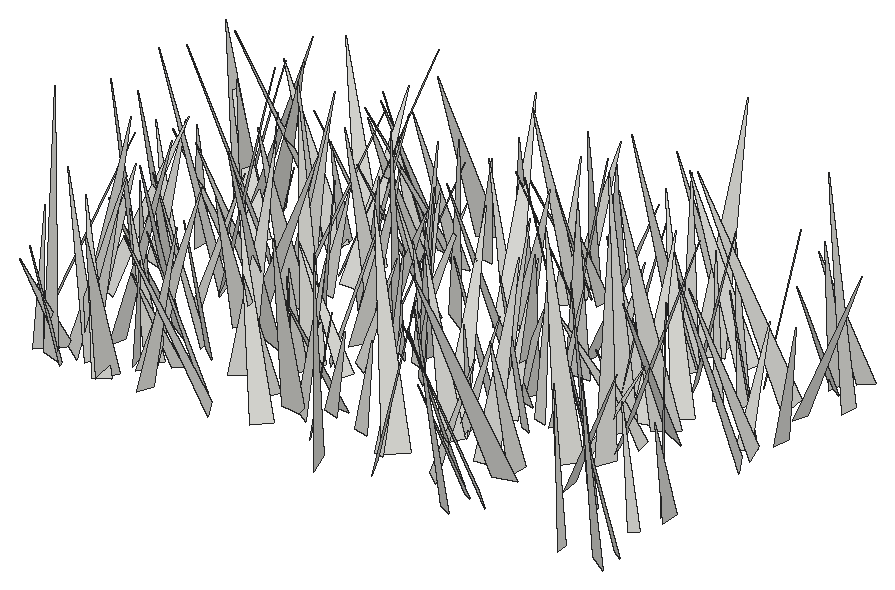
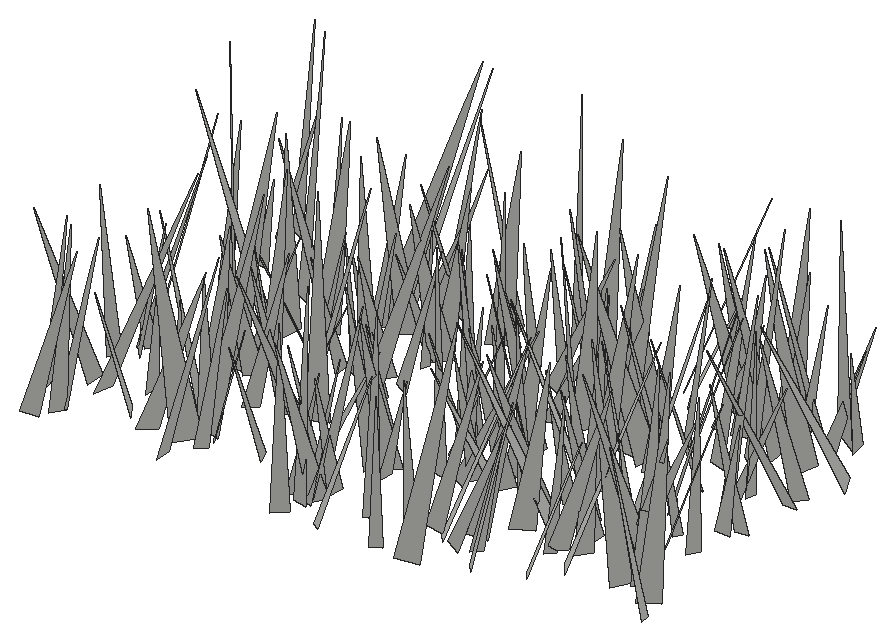
# SketchUp Ruby script. Lengths in inches.
U = 1.inch
M = Sketchup.active_model
def pt(a) = Geom::Point3d.new(a.map { |v| v * U })
def face(e, loops, mat)
  f = e.add_face(loops[0].map { |a| pt(a) })
  loops[1..].each { |l| e.add_face(l.map { |a| pt(a) }).erase! }
  f.material = f.back_material = mat if mat
  f
end
# faces: each face lists its corners as indices into pts; further lists are holes
def faces(e, pts, list, mat = nil) = list.each { |f| face(e, (f[0].is_a?(Array) ? f : [f]).map { |l| l.map { |i| pts[i] } }, mat) }
# xy, xz, yz: faces in a plane at the given z, y or x. An outline is a flat list of corners, or four numbers for a rectangle; further outlines are holes
def ring(l) = l.size == 4 ? [[l[0], l[1]], [l[2], l[1]], [l[2], l[3]], [l[0], l[3]]] : l.each_slice(2).to_a
def flat(e, list, mat, &to3) = list.each { |f| face(e, (f[0].is_a?(Array) ? f : [f]).map { |l| ring(l).map { |u, v| to3.(u, v) } }, mat) }
def xy(e, z, list, mat = nil) = flat(e, list, mat) { |x, y| [x, y, z] }
def xz(e, y, list, mat = nil) = flat(e, list, mat) { |x, z| [x, y, z] }
def yz(e, x, list, mat = nil) = flat(e, list, mat) { |y, z| [x, y, z] }
def lines(e, pts, list) = list.each { |a, b| e.add_line(pt(pts[a]), pt(pts[b])) }
# prism: a flat outline (further loops are holes) pulled along v
def prism(e, loops, v, mat = nil)
  f = face(e, loops, mat); d = Geom::Vector3d.new(v.map { |x| x * U })
  f.pushpull(f.normal.samedirection?(d) ? d.length : -d.length)
end
def box(e, o, s, mat = nil) = prism(e, [[o, [o[0] + s[0], o[1], o[2]], [o[0] + s[0], o[1] + s[1], o[2]], [o[0], o[1] + s[1], o[2]]]], [0, 0, s[2]], mat)
def at(x, y, z, deg = 0) = Geom::Transformation.translation(pt([x, y, z])) * Geom::Transformation.rotation(ORIGIN, Z_AXIS, deg.degrees)
def axes(o, x, y, z) = Geom::Transformation.new([*x, 0, *y, 0, *z, 0, *pt(o).to_a, 1])
def part(name) = M.definitions.add(name)
# library, detail: a bought-in or finely detailed component or shape, given as its bounding box
def library(name, o, s) = part(name).tap { |d| box(d.entities, o, s) }
def detail(e, o, s) = box(e.add_group.entities, o, s)
def put(e, d, t, mat = nil) = e.add_instance(d, t).tap { |i| i.material = mat if mat }
def group(e, t, mat = nil) = e.add_group.tap { |g| g.transformation = t; g.material = mat if mat }.entities
root = M.entities
c1 = part("fur_instance\#9")
p = [[0.8125,0,1.79],[0.67,-0.02,1.48],[0,-0.11,0],[0,0.11,0]]
faces(c1.entities,p,[[0,1,2,3]])
put(root,c1,axes([512.81,56.03,-21.66],[4.57924,-4.33247,0.58798],[-4.22206,-4.60304,-1.03525],[-1.13589,-0.35667,6.21836]))
put(root,c1,axes([519.8125,56.62,-21.66],[-5.72076,-3.26575,0.35826],[-3.1922,5.6955,0.94426],[0.77675,-0.64548,6.51924]))
put(root,c1,axes([528.72,55.54,-21.66],[6.72646,1.81373,2.96578],[2.30607,-7.16166,-0.85049],[-2.60144,-1.65881,6.91459]))
put(root,c1,axes([538.63,58.125,-21.66],[-4.50054,-5.78959,0.45114],[-5.68851,4.51005,1.13049],[1.1678,-0.3432,7.24542]))
put(root,c1,axes([548.48,56.47,-21.66],[-3.10043,-5.65859,2.0595],[-5.81568,3.41455,0.62657],[1.56175,1.48157,6.42182]))
put(root,c1,axes([508.82,57.23,-21.66],[1.51991,-3.61395,0.26794],[-3.4425,-1.53065,-1.11749],[-1.13207,-0.1975,3.75792]))
put(root,c1,axes([509.875,55.41,-21.66],[-3.12705,-1.8127,0.50032],[-1.87769,2.95706,-1.02213],[-0.10232,1.13341,3.46693]))
put(root,c1,axes([537.6875,55.89,-21.66],[-3.61019,-4.99925,2.09321],[-5.40705,3.49453,-0.97958],[0.37125,2.28107,6.08822]))
put(root,c1,axes([512.74,55.59,-21.66],[-2.01026,5.06538,1.49078],[5.275,1.85579,0.80751],[-0.23431,-1.67916,5.38954]))
put(root,c1,axes([515.45,56.19,-21.66],[5.24089,-0.83273,1.62957],[-1.05437,-5.41429,0.62423],[-1.49573,0.89885,5.2698]))
put(root,c1,axes([531.47,57.24,-21.66],[5.91305,2.63208,1.30513],[2.84881,-5.85376,-1.10147],[-0.71801,-1.54954,6.37799]))
put(root,c1,axes([508.86,55.72,-21.66],[2.99088,7.34321,2.70362],[7.47912,-3.53374,1.32409],[-2.30112,-1.94104,7.81761]))
put(root,c1,axes([545.77,56.53,-21.66],[-4.75488,-0.89522,1.48594],[-1.16705,4.85843,-0.80746],[1.28353,1.10117,4.77057]))
put(root,c1,axes([537.71,57.92,-21.66],[-2.11494,-3.26023,0.3236],[-3.25153,2.04149,-0.68318],[-0.40176,0.64034,3.82562]))
put(root,c1,axes([507.64,56.04,-21.66],[-4.10668,0.43412,1.0008],[0.12519,4.05996,-1.24738],[1.0837,1.17608,3.93666]))
put(root,c1,axes([509.49,56.92,-21.66],[3.29943,5.39851,1.49465],[5.593,-3.07886,-1.22601],[0.31023,-1.9081,6.20701]))
put(root,c1,axes([523.73,59.47,-21.66],[0.64901,-7.30772,0.94418],[-7.33385,-0.54888,0.79295],[0.71332,1.00569,7.2935]))
put(root,c1,axes([548.75,57.91,-21.66],[-3.27995,-3.84872,1.10692],[-4.00472,3.15616,-0.89264],[0.01123,1.42196,4.97734]))
put(root,c1,axes([513.13,58.27,-21.66],[3.69206,0.52175,1.19179],[0.74035,-3.79133,-0.63373],[-1.0698,-0.8231,3.6745]))
put(root,c1,axes([518.68,57.78,-21.66],[-4.50374,-2.5863,0.2222],[-2.55985,4.35118,-1.23954],[-0.43072,1.18335,5.04343]))
put(root,c1,axes([510.92,56.93,-21.66],[-5.72971,0.10944,0.75393],[-0.02545,5.68949,-1.01935],[0.7614,1.01378,5.63937]))
put(root,c1,axes([538.15,60.84,-21.66],[0.33917,-8.30019,0.61155],[-8.21231,-0.43312,-1.32383],[-1.35096,0.54903,8.20095]))
put(root,c1,axes([536.55,58.9,-21.66],[-2.94659,-4.28728,0.79485],[-4.35538,2.84813,-0.78348],[-0.2081,1.09651,5.14289]))
put(root,c1,axes([523.21,57.18,-21.66],[-3.60307,5.2202,0.86904],[5.28801,3.51043,0.83765],[-0.20649,-1.18922,6.28736]))
put(root,c1,axes([515.35,59.3125,-21.66],[0.6602,-3.48398,0.63366],[-3.31771,-0.83389,-1.12823],[-1.23791,0.37685,3.36171]))
put(root,c1,axes([513.87,59.01,-21.66],[2.18387,-4.44969,1.85832],[-4.59717,-2.53702,-0.67228],[-1.45572,1.33648,4.91091]))
put(root,c1,axes([526.45,57.6,-21.66],[2.93854,2.24557,1.05284],[2.03507,-3.11619,0.96641],[-1.41759,0.18132,3.56983]))
put(root,c1,axes([514.12,57.95,-21.66],[6.01682,-1.89651,1.60783],[-2.22,-5.99358,1.23799],[-1.11958,1.69241,6.18597]))
put(root,c1,axes([534.85,58.36,-21.66],[2.48119,3.58815,0.88423],[3.68479,-2.32113,-0.92071],[0.2811,-1.24521,4.2642]))
put(root,c1,axes([521.6,60.16,-21.66],[3.25434,-3.10316,1.28908],[-2.93626,-3.49873,-1.00964],[-1.63392,0.10675,4.38189]))
put(root,c1,axes([524.39,59.36,-21.66],[2.41252,4.65389,1.89869],[5.02303,-2.30836,-0.72433],[-0.1815,-2.02404,5.19175]))
put(root,c1,axes([528.28,59.95,-21.66],[0.50859,-3.54434,0.97529],[-3.61365,-0.30136,0.78924],[0.67458,1.05784,3.49258]))
put(root,c1,axes([525.55,60.61,-21.66],[0.50493,-3.90237,0.56248],[-3.75126,-0.30094,1.27958],[1.21364,0.69337,3.72104]))
put(root,c1,axes([530.68,58.56,-21.66],[1.32341,3.79294,0.4756],[3.74321,-1.38791,0.65276],[-0.77522,-0.22654,3.9638]))
put(root,c1,axes([525.92,61.32,-21.66],[-1.33885,-4.31341,0.19295],[-4.24788,1.27969,-0.86785],[-0.77346,0.43835,4.43226]))
put(root,c1,axes([531.43,59.28,-21.66],[-4.74257,5.72398,1.5327],[5.90767,4.72004,0.65254],[0.46105,-1.60076,7.40474]))
put(root,c1,axes([510.79,59.47,-21.66],[6.83211,0.09479,1.62922],[-0.11306,-6.96812,0.87954],[-1.62805,0.88169,6.77592]))
put(root,c1,axes([508.46,59.79,-21.66],[6.64236,-2.17739,2.19825],[-2.53423,-6.81539,0.90685],[-1.77512,1.5823,6.93106]))
put(root,c1,axes([512.82,62.5625,-21.66],[-2.64137,-6.46023,1.04071],[-6.35863,2.79897,1.23619],[1.54452,0.47506,6.86901]))
put(root,c1,axes([515.76,61.64,-21.66],[-2.72161,-4.19987,1.18368],[-4.18397,2.90781,0.69726],[1.23872,0.59401,4.95579]))
put(root,c1,axes([538.14,61.98,-21.66],[-4.48343,0.78051,2.64752],[1.64873,4.80743,1.37477],[2.21365,-1.99978,4.33824]))
put(root,c1,axes([543.55,62.14,-21.66],[-3.953,-6.85404,2.35159],[-6.87911,4.39144,1.23577],[2.27722,1.36799,7.81517]))
put(root,c1,axes([522.89,60.23,-21.66],[-3.3024,-1.44134,1.34219],[-1.74105,3.36144,-0.674],[0.92071,1.18661,3.53964]))
put(root,c1,axes([511.37,61.33,-21.66],[-4.43723,-6.45792,2.6794],[-6.95056,4.4181,-0.86196],[0.75734,2.71083,7.78786]))
put(root,c1,axes([548.45,63.11,-21.66],[4.29129,-1.7599,0.57931],[-1.53313,-4.1935,-1.38278],[-1.04037,-1.07949,4.42723]))
put(root,c1,axes([547.8,60.65,-21.66],[-0.43735,3.78387,0.74816],[3.7266,0.2203,1.06426],[-0.99494,-0.83814,3.65736]))
put(root,c1,axes([505.51,59.7,-21.66],[5.65943,2.62486,0.30549],[2.50558,-5.55953,1.3513],[-0.8398,1.10185,6.0904]))
put(root,c1,axes([541.65,62.45,-21.66],[5.27208,0.02621,0.0042],[0.02652,-5.23568,-0.61848],[-0.0011,-0.61849,5.23574]))
put(root,c1,axes([518.01,64.71,-21.66],[-1.4202,-8.16889,0.91065],[-8.13373,1.52988,1.03868],[1.18423,0.71114,8.22611]))
put(root,c1,axes([514.89,62.27,-21.66],[-5.1041,-1.8904,0.52095],[-1.9461,5.06157,-0.70004],[0.24022,0.83889,5.39772]))
put(root,c1,axes([521.18,63.26,-21.66],[3.43553,-2.13589,0.95207],[-2.02418,-3.56342,-0.68999],[-1.17096,-0.10667,3.98608]))
put(root,c1,axes([536.22,61.57,-21.66],[-1.99924,6.11191,2.2816],[6.3463,2.375,-0.80119],[1.51181,-1.88733,6.38047]))
put(root,c1,axes([518.68,60.92,-21.66],[5.55139,-3.03279,3.66915],[-4.09539,-5.91606,1.30628],[-2.42657,3.04644,6.18946]))
put(root,c1,axes([533.04,62.48,-21.66],[-4.86777,3.35697,1.6535],[3.6105,4.92638,0.62739],[0.98366,-1.46972,5.8797]))
put(root,c1,axes([506.51,62.82,-21.66],[2.49544,-4.2024,1.5625],[-4.46283,-2.15679,1.32672],[0.42981,2.0042,4.70396]))
put(root,c1,axes([547.34,63.79,-21.66],[6.08028,3.66314,2.96745],[4.34842,-6.22849,-1.22118],[-1.82087,-2.64225,6.99265]))
put(root,c1,axes([508.99,64.21,-21.66],[4.7247,0.27251,1.48983],[0.66278,-4.76043,-1.23114],[-1.36183,-1.37139,4.56961]))
put(root,c1,axes([533.07,63.99,-21.66],[3.93197,-0.07434,1.3447],[0.21137,-4.06439,-0.84276],[-1.33006,-0.86567,3.84131]))
put(root,c1,axes([515.14,65.55,-21.66],[4.0127,-3.86264,0.72099],[-3.71726,-4.06564,-1.09277],[-1.27351,-0.30356,5.46147]))
put(root,c1,axes([509.64,64.81,-21.66],[-1.12963,-3.6746,0.26296],[-3.62855,1.06225,-0.74377],[-0.63679,0.46567,3.77168]))
put(root,c1,axes([533.15,63.1,-21.66],[3.71678,-0.58843,1.31141],[-0.99782,-3.67326,1.17982],[-1.0346,1.42876,3.57333]))
put(root,c1,axes([523.51,64.55,-21.66],[-3.19624,2.75407,0.40141],[2.73336,2.9911,1.24258],[-0.52417,-1.19599,4.03198]))
put(root,c1,axes([539.93,64.58,-21.66],[-5.03128,5.10175,2.45438],[5.52933,5.13327,0.66454],[1.21582,-2.23324,7.13442]))
put(root,c1,axes([516.28,64.61,-21.66],[6.91635,-1.96319,0.7746],[-2.05636,-6.86586,0.95992],[-0.47486,1.1384,7.12521]))
put(root,c1,axes([532.75,62.86,-21.66],[-3.90742,5.66938,0.63215],[5.60395,3.95813,-0.85923],[1.06639,-0.02677,6.83166]))
put(root,c1,axes([521.38,64.19,-21.66],[-7.28379,2.71503,1.56111],[2.64145,7.44897,-0.63058],[1.68261,0.05921,7.74773]))
put(root,c1,axes([520.37,66.06,-21.66],[5.81902,2.09502,1.94943],[2.48849,-5.88572,-1.1028],[-1.4131,-1.7377,6.08555]))
put(root,c1,axes([506.48,63.76,-21.66],[1.55452,5.85258,0.28483],[5.77094,-1.47817,-1.12324],[1.01494,-0.55917,5.95042]))
put(root,c1,axes([539.57,65.29,-21.66],[1.87721,3.55983,2.07479],[3.45548,-2.60202,1.33802],[-2.2443,-1.02868,3.79553]))
put(root,c1,axes([511.88,65.3125,-21.66],[2.7927,4.03544,0.85961],[4.11922,-2.66751,-0.85986],[0.23622,-1.19268,4.83163]))
put(root,c1,axes([508.38,67.39,-21.66],[-2.6676,-6.3456,1.58153],[-6.4273,2.85927,0.63121],[1.20736,1.20081,6.85451]))
put(root,c1,axes([535.49,66.06,-21.66],[-2.59622,-3.87524,1.56211],[-4.17566,2.47102,-0.8099],[0.14666,1.75346,4.59368]))
put(root,c1,axes([523.5,65.8125,-21.66],[1.6531,3.56586,0.9383],[3.65871,-1.45863,-0.90264],[0.45784,-1.21883,3.82535]))
put(root,c1,axes([532.53,66.89,-21.66],[-2.18314,-4.32344,1.23175],[-4.48368,1.99494,-0.94459],[-0.32548,1.51774,4.75036]))
put(root,c1,axes([521.85,65.16,-21.66],[3.70568,3.40586,0.49894],[3.35111,-3.73706,0.62078],[-0.78668,0.12425,4.99466]))
put(root,c1,axes([541.56,65.85,-21.66],[-6.82221,1.72842,2.33339],[1.55801,7.20655,-0.7829],[2.45045,0.23004,6.99407]))
put(root,c1,axes([539.97,66.35,-21.66],[2.36408,2.77163,0.06713],[2.67068,-2.25294,-1.03299],[0.74428,-0.71945,3.49339]))
put(root,c1,axes([533.52,68.54,-21.66],[-2.92587,-7.18113,1.16279],[-7.26033,2.80394,-0.95233],[-0.45638,1.43204,7.69561]))
put(root,c1,axes([533.1875,69.09,-21.66],[6.03142,-3.81553,0.06105],[-3.78285,-5.99326,-0.84318],[-0.50203,-0.68018,7.08699]))
put(root,c1,axes([516.45,69.05,-21.66],[2.5513,-6.67742,1.15565],[-6.68995,-2.67869,-0.70836],[-1.08074,0.81812,7.11304]))
put(root,c1,axes([525.87,69.25,-21.66],[5.72206,-2.67718,0.30846],[-2.55509,-5.6197,-1.37653],[-0.85672,-1.12072,6.16558]))
put(root,c1,axes([525.14,66.66,-21.66],[-3.53887,0.08812,1.47041],[-0.2173,3.75324,-0.74791],[1.45693,0.77383,3.46005]))
put(root,c1,axes([541.94,68.82,-21.66],[-3.71284,-0.24914,0.82183],[0.046,3.58403,1.29433],[0.85753,-1.27095,3.48884]))
put(root,c1,axes([527.2,66.8,-21.66],[3.68214,4.39884,2.0354],[4.4735,-4.06815,0.69917],[-1.86561,-1.07294,5.69378]))
put(root,c1,axes([542.73,70.57,-21.66],[-1.67702,-6.45132,0.05531],[-6.32349,1.655,1.30744],[1.27907,-0.27646,6.53625]))
put(root,c1,axes([532.82,68.54,-21.66],[2.13927,-3.81253,0.27989],[-3.71667,-1.99926,1.17453],[0.89447,0.81104,4.21098]))
put(root,c1,axes([524.15,68.61,-21.66],[3.79237,5.90894,3.79832],[6.9076,-3.92109,-0.79686],[-1.27587,-3.6653,6.97586]))
put(root,c1,axes([533.98,66.38,-21.66],[-3.10832,3.75001,0.92239],[3.63037,3.24121,-0.94342],[1.31674,-0.08395,4.77852]))
put(root,c1,axes([511.85,67.94,-21.66],[-7.0839,-2.86843,1.00142],[-2.98784,7.03787,-0.97651],[0.55097,1.28563,7.57997]))
put(root,c1,axes([540.91,68.01,-21.66],[7.89024,2.57718,0.73013],[2.64489,-7.85516,-0.85554],[-0.42369,-1.04189,8.25626]))
put(root,c1,axes([535.51,67.33,-21.66],[1.56469,4.5597,1.40699],[4.65343,-1.78584,0.61247],[-1.05645,-1.11294,4.78163]))
put(root,c1,axes([521.78,67.87,-21.66],[5.79665,-1.91222,1.6292],[-2.17494,-5.87047,0.84811],[-1.25719,1.33905,6.04471]))
put(root,c1,axes([506.71,67.9,-21.66],[0.82444,4.69785,1.50621],[4.90559,-0.61872,-0.75536],[0.52313,-1.60174,4.70945]))
put(root,c1,axes([536.58,67.36,-21.66],[-4.01234,0.85775,1.7856],[0.34464,4.27421,-1.27879],[1.95072,1.00913,3.89863]))
put(root,c1,axes([547.68,70.55,-21.66],[-5.81163,-3.8947,1.27527],[-3.71182,5.94036,1.22659],[1.73708,-0.33677,6.88761]))
put(root,c1,axes([525.62,69.62,-21.66],[3.23004,-2.47849,1.2151],[-2.38486,-3.44753,-0.69249],[-1.3899,0.15559,4.01205]))
put(root,c1,axes([513.48,69.64,-21.66],[4.61843,1.91697,0.98697],[2.11588,-4.47821,-1.2031],[-0.41467,-1.49987,4.85358]))
put(root,c1,axes([507.57,68.6,-21.66],[-1.66438,3.94539,0.96796],[4.04045,1.49913,0.83702],[-0.42169,-1.20819,4.19948]))
put(root,c1,axes([526.01,68.07,-21.66],[2.58836,6.22661,1.98748],[6.38761,-2.86286,0.6503],[-1.38536,-1.56644,6.71174]))
put(root,c1,axes([511.66,67.93,-21.66],[6.24718,3.3719,1.68528],[3.2403,-6.4703,0.93425],[-1.92623,0.05148,7.03734]))
put(root,c1,axes([536.6875,69.58,-21.66],[-5.72763,-4.55632,1.57593],[-4.80185,5.61014,-1.23206],[0.43111,1.95337,7.21442]))
put(root,c1,axes([509.44,70.34,-21.66],[3.62629,-0.3933,0.08931],[-0.3696,-3.56406,-0.68808],[-0.16141,-0.67481,3.58206]))
put(root,c1,axes([520.99,70.77,-21.66],[1.6386,-6.2759,2.07036],[-6.47654,-1.94928,-0.78297],[-1.31443,1.78093,6.43885]))
put(root,c1,axes([541.84,71.04,-21.66],[2.92408,-7.38877,2.72238],[-7.56214,-3.44459,-1.22649],[-2.19528,2.02396,7.85111]))
put(root,c1,axes([511.32,70.93,-21.66],[-0.67131,-4.1889,0.93111],[-4.10147,0.34927,-1.38579],[-1.26165,1.09345,4.00962]))
put(root,c1,axes([547.5,72.07,-21.66],[-5.8236,-1.97497,1.08531],[-1.72724,5.8434,1.36532],[1.44743,-0.9731,5.99589]))
put(root,c1,axes([509.05,72.01,-21.66],[-4.05728,-2.523,0.42943],[-2.40041,4.03064,1.00168],[0.88766,-0.63233,4.67158]))
put(root,c1,axes([511.47,72.61,-21.66],[-5.81753,-5.50464,0.89808],[-5.45533,5.88597,0.73893],[1.16061,0.07452,7.97488]))
put(root,c1,axes([507.45,71.42,-21.66],[4.3427,-1.50818,1.19732],[-1.3579,-4.49272,-0.73402],[-1.36538,-0.32877,4.53816]))
put(root,c1,axes([540.08,69.5625,-21.66],[-7.50799,1.69583,1.59774],[1.55933,7.66276,-0.80567],[1.73121,0.45255,7.65484]))
put(root,c1,axes([525.82,70.52,-21.66],[-5.12979,-1.0122,0.11272],[-1.018,5.07872,-0.72273],[-0.03042,0.73083,5.17851]))
put(root,c1,axes([538.33,71.1,-21.66],[3.90059,1.73334,0.99556],[1.91928,-3.85762,-0.80331],[-0.55855,-1.15086,4.19211]))
put(root,c1,axes([516.6,71.29,-21.66],[-0.37702,3.57753,2.02822],[3.88687,0.97529,-0.99777],[1.34335,-1.81786,3.4562]))
put(root,c1,axes([520.51,72.17,-21.66],[3.4493,-3.36014,0.02886],[-3.29462,-3.37365,0.97621],[0.66096,0.719,4.71542]))
put(root,c1,axes([535.66,73.01,-21.66],[-3.34335,-1.51871,0.13226],[-1.40215,3.18862,1.16988],[0.59829,-1.01398,3.48078]))
put(root,c1,axes([533.93,72.84,-21.66],[1.85268,-6.56464,1.39244],[-6.70428,-1.74747,0.68181],[0.2934,1.52239,6.78691]))
put(root,c1,axes([518.4,73.18,-21.66],[5.40312,-1.02873,0.51523],[-0.87968,-5.28821,-1.33359],[-0.74156,-1.2223,5.33606]))
put(root,c1,axes([514.91,71.23,-21.66],[6.15209,3.35933,0.33959],[3.37614,-6.1107,-0.71393],[0.04606,-0.78923,6.97306]))
put(root,c1,axes([523.08,73.36,-21.66],[-1.88046,-5.21634,0.33238],[-5.10911,1.75978,-1.28722],[-1.10347,0.74146,5.39346]))
put(root,c1,axes([518.49,71.84,-21.66],[5.36031,4.39922,1.5205],[4.6383,-5.24227,-1.18439],[-0.38885,-1.88772,6.83252]))
put(root,c1,axes([530.55,70.43,-21.66],[1.48106,4.37962,0.44895],[4.22706,-1.54701,1.14671],[-1.23071,-0.04293,4.4788]))
put(root,c1,axes([524.4,73.45,-21.66],[-2.31612,-6.1908,2.36322],[-6.27799,2.85121,1.3163],[2.12077,1.67923,6.47748]))
put(root,c1,axes([522.84,72.18,-21.66],[2.35379,3.88662,0.95748],[3.9563,-2.09005,-1.24191],[0.60851,-1.44527,4.3708]))
put(root,c1,axes([514.25,72.32,-21.66],[4.29417,-2.87763,1.75823],[-3.19183,-4.38696,0.6155],[-1.08829,1.5119,5.13243]))
put(root,c1,axes([540.23,70.82,-21.66],[-3.17134,4.85922,0.78552],[4.77597,3.26378,-0.90795],[1.19131,-0.14895,5.73106]))
put(root,c1,axes([546.72,72.03,-21.66],[-2.21972,3.26489,1.22418],[3.2229,2.47495,-0.75684],[1.3308,-0.54808,3.87477]))
put(root,c1,axes([547.09,72.82,-21.66],[2.56501,3.25674,2.5986],[3.3721,-3.41499,0.95138],[-2.44704,-1.29222,4.03491]))
put(root,c1,axes([547.91,74.03,-21.66],[4.83385,-1.43847,0.54232],[-1.36908,-4.84202,-0.64023],[-0.69925,-0.46374,5.00254]))
put(root,c1,axes([522.52,72.52,-21.66],[-2.57998,2.99071,1.64125],[3.02202,2.95835,-0.64026],[1.58287,-0.77341,3.89753]))
put(root,c1,axes([538,73.875,-21.66],[-4.52682,2.09063,1.69581],[2.46981,4.54531,0.98938],[1.07078,-1.64562,4.88712]))
put(root,c1,axes([535.84,73.3,-21.66],[1.71183,-4.04593,1.56999],[-4.29437,-1.33542,1.2409],[0.62675,1.9005,4.21427]))
put(root,c1,axes([507.27,76.26,-21.66],[4.70982,-4.44224,0.12242],[-4.38661,-4.67586,-0.90827],[-0.71149,-0.57769,6.41023]))
put(root,c1,axes([541.74,72.7,-21.66],[-2.77056,6.19265,0.76015],[6.19361,2.62958,1.15202],[-0.75223,-1.15721,6.68563]))
put(root,c1,axes([512.31,75.42,-21.66],[5.42089,-2.3865,1.81758],[-2.19868,-5.71457,-0.94576],[-2.04078,-0.18248,5.84696]))
put(root,c1,axes([521.05,72.53,-21.66],[4.24517,2.47398,0.29086],[2.34061,-4.15824,1.20716],[-0.85248,0.90284,4.76286]))
put(root,c1,axes([512.71,73.75,-21.66],[5.08359,-0.28901,1.82683],[-0.68576,-5.25683,1.07667],[-1.71772,1.24337,4.97667]))
put(root,c1,axes([527.8,75.3,-21.66],[3.51302,-4.23345,1.0034],[-4.35037,-3.40123,0.88101],[0.05668,1.33409,5.43021]))
put(root,c1,axes([509.77,73.875,-21.66],[-3.53792,4.34861,0.23075],[4.30519,3.44804,1.02808],[-0.65501,-0.82532,5.51093]))
put(root,c1,axes([517.29,72.82,-21.66],[-1.69129,6.09931,0.73665],[6.01995,1.79783,-1.06428],[1.22654,-0.41345,6.23934]))
put(root,c1,axes([513.87,76.52,-21.66],[4.34393,-1.36952,0.92271],[-1.07858,-4.31928,-1.3331],[-1.25046,-1.03195,4.35524]))
put(root,c1,axes([508.99,75.42,-21.66],[3.83115,1.46002,1.29175],[1.69697,-3.89964,-0.62537],[-0.95945,-1.06731,4.05194]))
put(root,c1,axes([512.04,77.45,-21.66],[-5.96811,-4.81477,0.42538],[-4.75156,5.96808,0.88657],[0.88638,-0.42578,7.61672]))
put(root,c1,axes([508.34,76.93,-21.66],[6.88515,-2.28469,0.18682],[-2.24647,-6.84269,-0.88939],[-0.45618,-0.78602,7.19959]))
put(root,c1,axes([508.27,74.44,-21.66],[6.55283,1.12937,1.12544],[0.97488,-6.60494,0.95181],[-1.26162,0.76214,6.58096]))
put(root,c1,axes([518.27,77.71,-21.66],[1.50349,-5.86365,0.5049],[-5.82358,-1.55753,-0.74685],[-0.85041,0.2992,6.00709]))
put(root,c1,axes([540.07,75.82,-21.66],[5.73054,2.09287,1.0832],[2.24178,-5.71944,-0.8093],[-0.7265,-1.14039,6.04684]))
put(root,c1,axes([513.75,75.98,-21.66],[-5.32926,2.77314,1.19327],[2.9808,5.21718,1.1879],[0.47858,-1.6143,5.88899]))
put(root,c1,axes([505.83,77.55,-21.66],[4.78165,-4.93816,1.39024],[-4.88475,-4.96331,-0.82896],[-1.56762,0.40313,6.82367]))
put(root,c1,axes([533.17,74.86,-21.66],[5.62442,0.34622,0.61815],[0.22701,-5.5658,1.05184],[-0.67115,1.01884,5.53603]))
put(root,c1,axes([515.5625,74.09,-21.66],[6.75975,3.62956,0.52461],[3.54067,-6.74583,1.04905],[-0.95528,0.68056,7.60048]))
put(root,c1,axes([519.79,79.04,-21.66],[-4.86076,-4.47494,0.06756],[-4.36579,4.76306,1.38194],[0.98465,-0.972,6.46083]))
put(root,c1,axes([516.86,75.37,-21.66],[-4.60264,5.20733,0.96805],[5.29634,4.53648,0.77902],[0.04773,-1.24166,6.90606]))
put(root,c1,axes([545.83,77.65,-21.66],[-8.03194,-0.35365,0.82088],[-0.22203,7.97883,1.26494],[0.86581,-1.23463,7.93959]))
put(root,c1,axes([538.1,77.7,-21.66],[-1.48143,-7.59825,2.03928],[-7.84224,1.26126,-0.99758],[-0.62555,2.18232,7.67677]))
put(root,c1,axes([526.82,75.54,-21.66],[-4.67353,1.04438,0.03845],[1.02272,4.60667,-0.8165],[0.21505,0.78861,4.71868]))
put(root,c1,axes([543.59,75.95,-21.66],[-4.82421,0.67017,1.12309],[0.52178,4.9221,-0.69578],[1.19925,0.5543,4.82058]))
put(root,c1,axes([542.04,75.55,-21.66],[0.68638,4.30492,0.85677],[4.11958,-0.93113,1.37825],[-1.51508,-0.58153,4.13569]))
put(root,c1,axes([527.17,74.67,-21.66],[-3.85678,5.81728,0.33644],[5.7739,3.8696,-0.71896],[0.78484,0.11882,6.94252]))
put(root,c1,axes([530.33,77.85,-21.66],[-3.6362,-3.51378,0.23491],[-3.4583,3.49912,-1.19165],[-0.6648,1.01649,4.91412]))
put(root,c1,axes([520.81,78.5,-21.66],[-0.18696,-5.47828,1.21386],[-5.53827,-0.01495,-0.92048],[-0.90141,1.22808,5.40363]))
put(root,c1,axes([546.94,76.99,-21.66],[5.55155,-0.72144,0.45458],[-0.77671,-5.51397,0.73462],[-0.35191,0.78896,5.54982]))
put(root,c1,axes([513.29,79.41,-21.66],[-3.4189,-2.83051,0.24342],[-2.77437,3.40847,0.66713],[0.61145,-0.36118,4.38812]))
put(root,c1,axes([537.24,79.375,-21.66],[4.28198,-1.79299,1.3249],[-1.43721,-4.41332,-1.32759],[-1.70429,-0.78312,4.44833]))
put(root,c1,axes([537.33,78.05,-21.66],[-3.51582,-2.14374,0.80605],[-2.26912,3.46073,-0.69338],[0.31056,1.01688,4.05904]))
put(root,c1,axes([524.47,79.75,-21.66],[-0.27546,-6.0552,1.07535],[-6.00995,0.49341,1.23885],[1.30474,0.99438,5.93351]))
put(root,c1,axes([538.68,77.18,-21.66],[-5.6137,1.8249,1.28834],[1.63706,5.7317,-0.98561],[1.51991,0.56669,5.82001]))
put(root,c1,axes([517.29,79,-21.66],[-3.50463,1.38607,1.3282],[1.66931,3.56562,0.68373],[0.94799,-1.15452,3.70623]))
put(root,c1,axes([504.83,79.14,-21.66],[4.88196,1.64498,0.71636],[1.77456,-4.73338,-1.22423],[-0.26474,-1.39349,5.00407]))
put(root,c1,axes([546.35,80.79,-21.66],[-1.70648,-4.83175,0.15849],[-4.67215,1.69151,1.26205],[1.24174,-0.27565,4.96639]))
put(root,c1,axes([518.73,79.41,-21.66],[-1.8038,-4.78632,0.84713],[-4.75617,1.55162,-1.36069],[-1.00264,1.25053,4.93062]))
put(root,c1,axes([529.75,80.41,-21.66],[2.79879,-2.29313,0.37979],[-2.08936,-2.74248,-1.16161],[-1.01846,-0.6755,3.42672]))
put(root,c1,axes([533.73,78.05,-21.66],[3.61402,1.40651,0.81578],[1.29809,-3.69316,0.61679],[-0.97915,0.29527,3.8287]))
put(root,c1,axes([528.375,79.71,-21.66],[-6.31827,-0.38458,1.65434],[-0.20418,6.49842,0.73085],[1.68614,-0.65417,6.28763]))
put(root,c1,axes([521.23,80.125,-21.66],[0.93641,-4.49496,0.58968],[-4.44892,-0.79539,1.00188],[0.87152,0.76939,4.48082]))
put(root,c1,axes([529.68,77.72,-21.66],[4.20978,2.5999,1.29958],[2.36123,-4.39284,1.13935],[-1.69498,0.33775,4.81493]))
put(root,c1,axes([528.42,80.68,-21.66],[-1.9531,-3.93926,0.49775],[-3.87343,2.01224,0.72636],[0.87298,0.11511,4.33645]))
put(root,c1,axes([516.32,80.81,-21.66],[-3.7934,-3.57067,0.95546],[-3.47781,3.9116,0.81037],[1.25196,0.04698,5.14615]))
put(root,c1,axes([541.03,79.6,-21.66],[-5.49496,2.98551,0.84144],[3.09795,5.36781,1.18541],[0.15494,-1.44541,6.14025]))
put(root,c1,axes([528.74,80.94,-21.66],[-1.97091,-5.99186,1.73382],[-5.97714,2.33419,1.27215],[1.7839,1.20092,6.17807]))
put(root,c1,axes([519.7,82.43,-21.66],[2.52782,-6.77606,0.30453],[-6.73549,-2.54598,-0.74076],[-0.80053,0.02468,7.19418]))
put(root,c1,axes([527.9,78.72,-21.66],[3.76541,-0.98312,2.37268],[-1.72485,-4.08783,1.04352],[-1.9029,1.75998,3.74912]))
put(root,c1,axes([546.32,81.22,-21.66],[5.03393,-2.19184,1.50174],[-1.99616,-5.24318,-0.96135],[-1.75349,-0.32355,5.40559]))
put(root,c1,axes([543.01,78.61,-21.66],[3.77893,2.89431,1.05154],[2.64296,-3.90266,1.24382],[-1.58036,0.3941,4.59459]))
put(root,c1,axes([538.375,81.5,-21.66],[-6.39849,-1.36399,1.46981],[-1.16574,6.52941,0.98452],[1.63152,-0.68393,6.46776]))
put(root,c1,axes([526.34,82.48,-21.66],[-3.05725,-3.63504,0.09512],[-3.51202,2.98398,1.15363],[0.94245,-0.67208,4.60753]))
put(root,c1,axes([548.6,79.37,-21.66],[-7.01031,-0.43579,1.43561],[-0.72042,6.99511,-1.39453],[1.31601,1.50792,6.88401]))
put(root,c1,axes([538.4,79.25,-21.66],[-4.94866,6.16749,2.69055],[6.18584,5.48419,-1.19385],[2.6481,-1.28527,7.81677]))
put(root,c1,axes([528.09,80.03,-21.66],[-2.58112,4.19595,2.18678],[4.13957,3.20902,-1.27135],[2.29171,-1.07069,4.75939]))
put(root,c1,axes([547.41,82.47,-21.66],[1.87791,-4.76016,0.94457],[-4.63856,-2.05833,-1.15104],[-1.42657,0.4266,4.98606]))
put(root,c1,axes([528.99,82.48,-21.66],[4.92449,-2.5321,0.51516],[-2.43841,-4.92066,-0.87679],[-0.85503,-0.55051,5.46748]))
put(root,c1,axes([522.125,82.23,-21.66],[0.84886,-4.32385,0.54485],[-4.30912,-0.7498,0.76315],[0.65118,0.6747,4.3398]))
